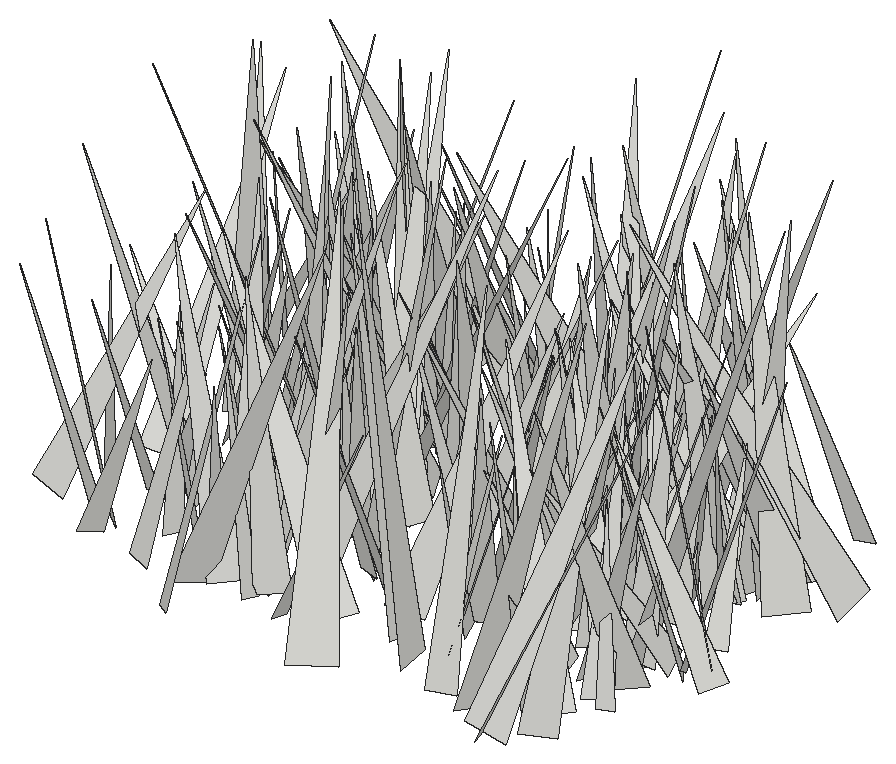
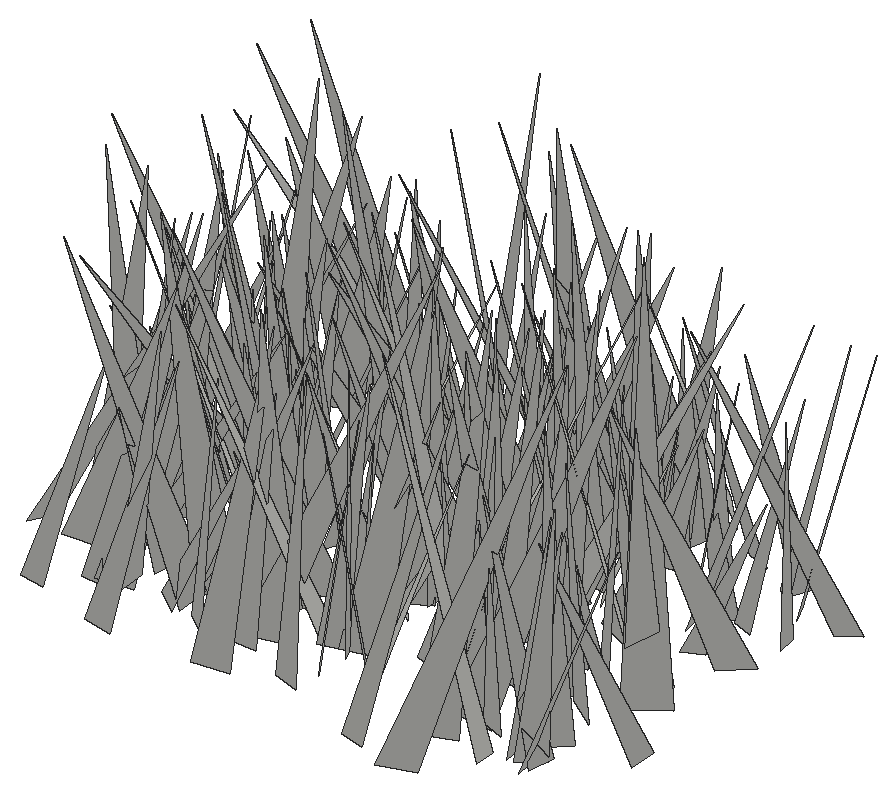
# SketchUp Ruby script. Lengths in inches.
U = 1.inch
M = Sketchup.active_model
def pt(a) = Geom::Point3d.new(a.map { |v| v * U })
def face(e, loops, mat)
  f = e.add_face(loops[0].map { |a| pt(a) })
  loops[1..].each { |l| e.add_face(l.map { |a| pt(a) }).erase! }
  f.material = f.back_material = mat if mat
  f
end
# faces: each face lists its corners as indices into pts; further lists are holes
def faces(e, pts, list, mat = nil) = list.each { |f| face(e, (f[0].is_a?(Array) ? f : [f]).map { |l| l.map { |i| pts[i] } }, mat) }
# xy, xz, yz: faces in a plane at the given z, y or x. An outline is a flat list of corners, or four numbers for a rectangle; further outlines are holes
def ring(l) = l.size == 4 ? [[l[0], l[1]], [l[2], l[1]], [l[2], l[3]], [l[0], l[3]]] : l.each_slice(2).to_a
def flat(e, list, mat, &to3) = list.each { |f| face(e, (f[0].is_a?(Array) ? f : [f]).map { |l| ring(l).map { |u, v| to3.(u, v) } }, mat) }
def xy(e, z, list, mat = nil) = flat(e, list, mat) { |x, y| [x, y, z] }
def xz(e, y, list, mat = nil) = flat(e, list, mat) { |x, z| [x, y, z] }
def yz(e, x, list, mat = nil) = flat(e, list, mat) { |y, z| [x, y, z] }
def lines(e, pts, list) = list.each { |a, b| e.add_line(pt(pts[a]), pt(pts[b])) }
# prism: a flat outline (further loops are holes) pulled along v
def prism(e, loops, v, mat = nil)
  f = face(e, loops, mat); d = Geom::Vector3d.new(v.map { |x| x * U })
  f.pushpull(f.normal.samedirection?(d) ? d.length : -d.length)
end
def box(e, o, s, mat = nil) = prism(e, [[o, [o[0] + s[0], o[1], o[2]], [o[0] + s[0], o[1] + s[1], o[2]], [o[0], o[1] + s[1], o[2]]]], [0, 0, s[2]], mat)
def at(x, y, z, deg = 0) = Geom::Transformation.translation(pt([x, y, z])) * Geom::Transformation.rotation(ORIGIN, Z_AXIS, deg.degrees)
def axes(o, x, y, z) = Geom::Transformation.new([*x, 0, *y, 0, *z, 0, *pt(o).to_a, 1])
def part(name) = M.definitions.add(name)
# library, detail: a bought-in or finely detailed component or shape, given as its bounding box
def library(name, o, s) = part(name).tap { |d| box(d.entities, o, s) }
def detail(e, o, s) = box(e.add_group.entities, o, s)
def put(e, d, t, mat = nil) = e.add_instance(d, t).tap { |i| i.material = mat if mat }
def group(e, t, mat = nil) = e.add_group.tap { |g| g.transformation = t; g.material = mat if mat }.entities
root = M.entities
c1 = part("fur_instance\#9")
p = [[0.8125,0,1.79],[0.67,-0.02,1.48],[0,-0.11,0],[0,0.11,0]]
faces(c1.entities,p,[[0,1,2,3]])
put(root,c1,axes([131.79,358.97,-27.1],[7.44072,-1.6859,2.03296],[-2.09272,-7.4711,1.46382],[-1.61112,1.91833,7.48758]))
put(root,c1,axes([133.125,357.88,-27.1],[-0.55252,7.61083,1.2014],[7.43516,0.84266,-1.91879],[2.02152,-1.01911,7.38568]))
put(root,c1,axes([134.1875,358.99,-27.1],[-5.16392,-1.1559,0.80889],[-1.35151,4.93357,-1.57791],[0.40477,1.72635,5.05098]))
put(root,c1,axes([125.68,357.83,-27.1],[-5.56313,6.05819,1.00831],[6.02083,5.64819,-0.71719],[1.2116,-0.25113,8.19364]))
put(root,c1,axes([114.08,360.4,-27.1],[3.45367,-2.54495,0.42724],[-2.57712,-3.36456,0.79082],[0.1334,0.88889,4.21654]))
put(root,c1,axes([123.74,360.28,-27.1],[6.28963,-0.96384,2.1084],[-1.07131,-6.61487,0.17192],[-2.05588,0.49827,6.36073]))
put(root,c1,axes([118.91,359.8,-27.1],[6.76451,-3.26106,1.25254],[-3.47694,-6.54929,1.72622],[-0.33809,2.1058,7.30844]))
put(root,c1,axes([128.125,360.22,-27.1],[-7.87878,-1.52664,2.20407],[-1.70967,8.13085,-0.47967],[2.06533,0.90687,8.01097]))
put(root,c1,axes([133.12,357.53,-27.1],[6.18332,3.30926,0.01495],[3.17233,-5.93637,1.96995],[-0.9422,1.73008,6.73082]))
put(root,c1,axes([122.71,359.79,-27.1],[3.9235,0.14114,0.37721],[0.06723,-3.8717,0.74932],[-0.3971,0.73898,3.85386]))
put(root,c1,axes([119.34,357.74,-27.1],[4.35483,5.04158,0.80125],[4.65214,-4.35304,2.10539],[-2.1017,0.81089,6.32055]))
put(root,c1,axes([118.79,361.35,-27.1],[3.85883,-1.0172,1.02296],[-0.87371,-3.97244,-0.65425],[-1.14794,-0.39587,3.93665]))
put(root,c1,axes([113.28,361.72,-27.1],[-4.38014,-2.49103,0.91186],[-2.44951,4.47381,0.4553],[1.01814,0.04674,5.01832]))
put(root,c1,axes([129.71,359.67,-27.1],[2.50571,3.8301,0.73521],[3.84486,-2.57244,0.29737],[-0.65369,-0.44905,4.56726]))
put(root,c1,axes([121.5625,360.86,-27.1],[-3.51075,4.42455,2.16586],[4.8357,3.60279,0.47842],[0.94002,-2.00904,5.62789]))
put(root,c1,axes([119.84,360.53,-27.1],[-3.34146,5.15286,1.47209],[5.35695,3.16362,1.08579],[-0.14849,-1.82317,6.0447]))
put(root,c1,axes([116.61,359.82,-27.1],[2.03381,4.83721,0.83738],[4.90479,-2.04045,-0.1258],[-0.20703,-0.82108,5.24587]))
put(root,c1,axes([121.15,360.2,-27.1],[-4.31173,0.11749,0.33288],[0.02447,4.16916,-1.1546],[0.35215,1.14887,4.15592]))
put(root,c1,axes([114.28,361.38,-27.1],[-4.01169,-3.78695,1.3287],[-4.00574,3.89344,-0.9976],[0.2459,1.64323,5.42581]))
put(root,c1,axes([125.25,362.83,-27.1],[-2.82637,-5.01502,0.69558],[-5.06125,2.81969,-0.23605],[0.13409,0.7222,5.75179]))
put(root,c1,axes([132.3,360.89,-27.1],[-3.8319,-0.08961,1.0116],[-0.27638,3.8917,-0.7022],[0.97723,0.7493,3.76807]))
put(root,c1,axes([134.18,360.33,-27.1],[-3.78417,5.30239,0.2634],[5.25954,3.70033,1.07214],[-0.72248,-0.83479,6.42541]))
put(root,c1,axes([124.35,360.86,-27.1],[-4.44973,5.42889,0.1833],[5.21151,4.19987,2.12315],[-1.53186,-1.48148,6.69068]))
put(root,c1,axes([135.0625,363.33,-27.1],[2.07945,-5.56592,1.40736],[-5.43571,-2.39045,-1.42237],[-1.84751,0.76846,5.76892]))
put(root,c1,axes([130.25,359.08,-27.1],[0.51601,7.02264,0.2402],[6.84431,-0.55684,1.57697],[-1.5908,-0.11784,6.86272]))
put(root,c1,axes([120.35,361.39,-27.1],[0.83525,-3.69964,2.10924],[-4.22949,-0.46947,0.8514],[0.49764,2.21949,3.69595]))
put(root,c1,axes([118.83,362.11,-27.1],[-2.76713,3.18046,1.2921],[3.43249,2.58898,0.97827],[0.05304,-1.61979,4.10065]))
put(root,c1,axes([134.68,358.78,-27.1],[-6.77077,3.15469,0.89527],[2.64884,6.47215,-2.77341],[1.93319,2.18084,6.93567]))
put(root,c1,axes([117.28,362.17,-27.1],[-3.57369,-1.9669,1.0397],[-2.0892,3.64317,-0.28897],[0.76478,0.76131,4.06896]))
put(root,c1,axes([128.33,363.02,-27.1],[-3.2792,-1.26365,1.37089],[-0.97388,3.52607,0.9207],[1.58988,-0.44645,3.3915]))
put(root,c1,axes([128.36,363.73,-27.1],[2.49567,-4.97649,0.70111],[-5.02561,-2.47346,0.33254],[-0.01412,0.77585,5.55727]))
put(root,c1,axes([120.59,361.31,-27.1],[4.03025,7.20792,1.49357],[7.34455,-3.82368,-1.36555],[0.49235,-1.96292,8.14446]))
put(root,c1,axes([126.84,361.29,-27.1],[-7.00273,-0.39667,0.95685],[-0.59042,6.90153,-1.45992],[0.85107,1.52402,6.86034]))
put(root,c1,axes([116.36,362.03,-27.1],[-3.76859,1.24193,1.36163],[1.17189,4.00702,-0.41131],[1.42236,-0.01087,3.94658]))
put(root,c1,axes([114.88,363.66,-27.1],[1.3305,-3.93215,0.09517],[-3.71952,-1.22514,1.38031],[1.27907,0.52755,3.91494]))
put(root,c1,axes([135.32,361.63,-27.1],[-0.19051,3.61425,0.52762],[3.57644,0.0773,0.76192],[-0.74175,-0.55561,3.53816]))
put(root,c1,axes([132.47,363.39,-27.1],[-4.25232,-1.15186,0.17503],[-1.13335,4.24309,0.38907],[0.27009,-0.33025,4.38835]))
put(root,c1,axes([114.16,363.74,-27.1],[-1.28236,-4.10189,0.60594],[-4.14572,1.27987,-0.10961],[0.07509,0.61118,4.29626]))
put(root,c1,axes([133.57,363.1,-27.1],[4.86131,-2.02952,0.59697],[-2.06386,-4.87843,0.22145],[-0.46454,0.43544,5.26329]))
put(root,c1,axes([119.67,361.91,-27.1],[-2.53684,6.34204,1.9532],[6.60869,2.60398,0.12835],[0.60133,-1.86275,6.82939]))
put(root,c1,axes([120.46,362.1,-27.1],[3.86814,-0.78573,1.02615],[-1.07279,-3.75781,1.16655],[-0.72076,1.37634,3.77081]))
put(root,c1,axes([135.16,365.58,-27.1],[-5.02387,-1.18033,0.42976],[-0.88594,4.58548,2.23734],[0.8905,-2.09699,4.65046]))
put(root,c1,axes([128.69,361.59,-27.1],[4.75922,3.00167,0.77273],[2.8511,-4.79497,1.06623],[-1.21588,0.50555,5.5248]))
put(root,c1,axes([128.02,364.64,-27.1],[6.9866,-0.46387,0.39437],[-0.38095,-6.874,-1.33651],[-0.47495,-1.31005,6.87325]))
put(root,c1,axes([111.05,361.9,-27.1],[0.65701,6.39206,0.99008],[6.12037,-0.29236,-2.17392],[2.09278,-1.15171,6.04683]))
put(root,c1,axes([134.65,362.01,-27.1],[-3.96377,3.38106,0.80717],[3.27975,4.04327,-0.83051],[1.15166,0.12228,5.14327]))
put(root,c1,axes([120.79,364.92,-27.1],[2.81621,-4.35059,0.38195],[-4.36621,-2.81499,0.12899],[-0.09891,0.39082,5.18093]))
put(root,c1,axes([112.28,363.67,-27.1],[3.8396,0.83392,1.68617],[0.96833,-4.16197,-0.14664],[-1.61273,-0.51356,3.92638]))
put(root,c1,axes([123.21,364,-27.1],[-3.81075,-5.76969,1.72606],[-6.01138,3.52106,-1.50194],[-0.36316,2.25903,6.74947]))
put(root,c1,axes([115.74,364.3,-27.1],[-6.60705,-1.5953,0.55499],[-1.61141,6.62494,-0.14037],[0.50631,0.26714,6.79547]))
put(root,c1,axes([135.77,365.24,-27.1],[-4.16981,-3.31895,0.85743],[-3.36405,4.22145,-0.01946],[0.65859,0.54939,5.32938]))
put(root,c1,axes([122.56,361.57,-27.1],[3.274,7.7332,0.0389],[7.72076,-3.26624,-0.49451],[0.44025,-0.22856,8.38313]))
put(root,c1,axes([130.0625,362.83,-27.1],[4.92859,0.75105,0.39032],[0.57555,-4.66461,1.7081],[-0.62062,1.63853,4.68375]))
put(root,c1,axes([130.85,365.08,-27.1],[4.88822,-0.89007,0.63341],[-0.87396,-4.92864,-0.18113],[-0.65546,-0.06625,4.96529]))
put(root,c1,axes([137.24,365.07,-27.1],[-3.88127,2.88585,0.74535],[2.95869,3.58243,1.53633],[-0.36036,-1.66913,4.58608]))
put(root,c1,axes([117.11,365.25,-27.1],[-3.35519,-0.75879,1.11745],[-0.66434,3.53232,0.40387],[1.17606,-0.1694,3.41613]))
put(root,c1,axes([122.875,364.34,-27.1],[4.94057,6.27292,2.28459],[6.62263,-4.9638,-0.69253],[-0.84236,-2.23369,7.95482]))
put(root,c1,axes([121.28,365.89,-27.1],[4.3252,-1.84495,1.08949],[-1.74272,-4.45705,-0.62914],[-1.2465,-0.1704,4.65998]))
put(root,c1,axes([119.76,364.64,-27.1],[-1.17344,-6.36654,3.3674],[-7.15717,1.41187,0.17527],[0.80444,3.27459,6.4714]))
put(root,c1,axes([133.66,363.99,-27.1],[-3.54308,4.52564,0.44169],[4.5332,3.47169,0.79207],[-0.35583,-0.83417,5.69276]))
put(root,c1,axes([119.19,364.98,-27.1],[-3.56795,-1.90054,0.20659],[-1.88749,3.43261,-1.0196],[-0.30353,0.99505,3.91187]))
put(root,c1,axes([121.06,365.91,-27.1],[3.12862,-2.29976,0.97047],[-2.27,-3.26853,-0.42753],[-1.03819,0.21622,3.85932]))
put(root,c1,axes([119.6,366.09,-27.1],[-2.97,-5.19915,0.68344],[-5.09037,2.66981,-1.8109],[-1.25951,1.46972,5.70725]))
put(root,c1,axes([134.15,364.83,-27.1],[-0.55684,5.82392,2.02647],[6.12632,0.75415,-0.48394],[0.70204,-1.96161,5.83043]))
put(root,c1,axes([126.51,365.66,-27.1],[-4.66446,-0.17714,0.77084],[-0.14932,4.72517,0.1823],[0.77671,-0.15541,4.66426]))
put(root,c1,axes([135.9,366.5625,-27.1],[4.20893,3.73459,3.7879],[4.59902,-4.98198,-0.19834],[-2.67289,-2.69131,5.62342]))
put(root,c1,axes([131.53,367.64,-27.1],[4.41778,-6.32124,1.65754],[-6.32459,-4.6393,-0.83587],[-1.6447,0.86086,7.66656]))
put(root,c1,axes([124.6,366.7,-27.1],[3.18493,-3.37138,0.77047],[-3.44968,-3.17103,0.3845],[-0.24394,0.82581,4.62191]))
put(root,c1,axes([132.14,364.63,-27.1],[-4.57761,1.25738,1.06742],[0.91701,4.55759,-1.43608],[1.37093,1.14988,4.52473]))
put(root,c1,axes([131.1,365.93,-27.1],[1.65832,3.59632,1.35209],[3.82471,-1.68517,-0.20869],[-0.36513,-1.31848,3.95475]))
put(root,c1,axes([125.84,362.64,-27.1],[-5.17652,4.83446,1.05401],[3.91261,4.93311,-3.41105],[3.02894,1.88989,6.20751]))
put(root,c1,axes([114.41,366.1,-27.1],[-3.16167,2.60611,0.16715],[2.5519,3.02748,1.0668],[-0.55458,-0.92652,3.956]))
put(root,c1,axes([118.93,368.58,-27.1],[7.2919,-1.58164,0.56037],[-1.39543,-7.10365,-1.89164],[-0.93186,-1.73896,7.21769]))
put(root,c1,axes([129.96,366.41,-27.1],[-5.05494,-2.22544,0.30278],[-2.23904,4.935,-1.10864],[-0.17591,1.1357,5.41072]))
put(root,c1,axes([127.45,368.08,-27.1],[-5.15654,-2.89646,0.02201],[-2.88562,5.14083,0.47427],[0.2514,-0.40276,5.89529]))
put(root,c1,axes([131.22,365.33,-27.1],[-1.86481,4.13252,0.34952],[4.14724,1.85655,0.17621],[-0.01744,-0.39104,4.53037]))
put(root,c1,axes([130.72,367.17,-27.1],[4.45339,-2.56263,0.11815],[-2.55046,-4.39735,0.75645],[0.27609,0.71411,5.08208]))
put(root,c1,axes([119.44,367.03,-27.1],[-6.03257,-5.76703,0.56772],[-5.59645,5.58532,-2.7307],[-1.50355,2.34912,7.8863]))
put(root,c1,axes([128.52,368.02,-27.1],[-4.47409,-0.55232,0.95951],[-0.288,4.43762,1.21151],[1.069,-1.11608,4.34221]))
put(root,c1,axes([119.45,366.52,-27.1],[5.54301,-4.89223,1.08245],[-4.92161,-5.01325,2.54471],[0.93987,2.60075,6.94141]))
put(root,c1,axes([132.03,368.08,-27.1],[-2.90046,-3.39812,1.38689],[-3.27993,3.19309,0.96417],[1.64705,0.37459,4.36237]))
put(root,c1,axes([133.33,366.18,-27.1],[-4.45117,0.87592,1.04433],[0.68712,4.52233,-0.86441],[1.17717,0.67238,4.45342]))
put(root,c1,axes([117.28,366.79,-27.1],[-0.49335,5.1966,1.87912],[5.02115,-0.36617,2.33091],[-2.30734,-1.90798,4.67065]))
put(root,c1,axes([134.33,364.45,-27.1],[7.79418,1.63756,2.08164],[0.8535,-7.67768,2.8441],[-2.50726,2.47704,7.43922]))
put(root,c1,axes([123.875,369.34,-27.1],[4.30968,-5.09044,0.61484],[-5.06109,-4.35201,-0.55619],[-0.82219,0.10671,6.64655]))
put(root,c1,axes([113.53,368.77,-27.1],[6.27835,0.76334,0.54412],[0.88551,-6.03847,-1.74618],[-0.30762,-1.80294,6.07875]))
put(root,c1,axes([116.91,369.44,-27.1],[-0.2881,-6.79413,1.19024],[-6.52945,0.65262,2.14482],[2.22333,1.03623,6.45314]))
put(root,c1,axes([130.15,368.46,-27.1],[-3.55733,-3.55392,1.20149],[-3.66341,3.64755,-0.05732],[0.80828,0.89081,5.02808]))
put(root,c1,axes([114.26,368.78,-27.1],[1.4923,-4.43759,0.64343],[-4.35505,-1.27294,1.3215],[1.06759,1.01025,4.49142]))
put(root,c1,axes([118.21,367.39,-27.1],[3.92442,2.27765,0.90763],[2.32456,-4.0011,-0.01041],[-0.77966,-0.46478,4.53747]))
put(root,c1,axes([129.31,368.47,-27.1],[1.81609,-4.28388,1.69446],[-4.45246,-2.09973,-0.53642],[-1.18256,1.32684,4.62191]))
put(root,c1,axes([131.38,366.43,-27.1],[7.46967,2.68884,2.29218],[2.3982,-7.79505,1.32883],[-2.59473,0.53597,7.82688]))
put(root,c1,axes([124.96,367.39,-27.1],[0.90877,4.85728,1.17196],[4.86719,-0.59112,-1.32422],[1.13009,-1.36012,4.76083]))
put(root,c1,axes([122.35,367.67,-27.1],[-5.92125,2.00992,1.02968],[2.02644,6.00419,-0.06686],[0.99676,-0.26678,6.25272]))
put(root,c1,axes([135.64,367.19,-27.1],[-2.23531,2.8422,0.49749],[2.78374,2.28983,-0.57415],[0.75919,-0.0278,3.57002]))
put(root,c1,axes([135.74,365.3,-27.1],[4.27823,3.00126,0.70858],[2.21616,-3.83495,2.86263],[-2.14435,2.02448,4.3722]))
put(root,c1,axes([131.73,367.75,-27.1],[5.13146,2.31605,0.71954],[2.33013,-5.17519,0.0403],[-0.67253,-0.25897,5.62978]))
put(root,c1,axes([121.19,370.19,-27.1],[-6.73685,-3.71008,0.0403],[-3.70619,6.73292,0.28887],[0.17463,-0.23362,7.68547]))
put(root,c1,axes([123.37,368.46,-27.1],[5.69837,-0.41307,2.53776],[-0.52377,-6.22748,0.16244],[-2.51724,0.36068,5.71101]))
put(root,c1,axes([133.03,369.15,-27.1],[4.02483,1.17033,1.17041],[1.40502,-4.04247,-0.78939],[-0.87491,-1.10794,4.11653]))
put(root,c1,axes([134.375,369.09,-27.1],[-3.74193,-1.93414,1.83822],[-1.95383,4.14237,0.38123],[1.81727,0.47108,4.19495]))
put(root,c1,axes([131.4,368.625,-27.1],[1.02394,3.35387,1.44831],[3.57422,-1.23084,0.32333],[-0.75567,-1.27715,3.49176]))
put(root,c1,axes([112.5625,366.07,-27.1],[-2.48989,6.58556,0.19317],[6.42005,2.47161,-1.51018],[1.47984,0.3578,6.87667]))
put(root,c1,axes([113.17,370.14,-27.1],[4.71718,-6.41333,2.08506],[-6.64537,-4.85367,0.10513],[-1.14777,1.74389,7.96063]))
put(root,c1,axes([113.81,369.82,-27.1],[4.65785,-0.69082,1.21899],[-0.53967,-4.78978,-0.65231],[-1.29303,-0.48941,4.6634]))
put(root,c1,axes([133.98,369.73,-27.1],[4.51203,-4.20905,2.90182],[-4.30887,-5.21386,-0.8628],[-2.75143,1.26279,6.10984]))
put(root,c1,axes([119.36,370,-27.1],[-4.57691,0.82768,1.57562],[1.18388,4.66198,0.99001],[1.32893,-1.30255,4.54457]))
put(root,c1,axes([115.57,369.44,-27.1],[-3.42106,-4.15596,2.05732],[-4.44833,3.66341,0.00339],[1.31032,1.58608,5.3829]))
put(root,c1,axes([133.96,370.01,-27.1],[0.76269,-3.95415,0.89534],[-4.04548,-0.80213,-0.09639],[-0.26648,0.86018,4.02588]))
put(root,c1,axes([114.61,370.36,-27.1],[5.46808,5.3055,1.78388],[5.41419,-4.38056,-3.56761],[1.42026,-3.72732,6.73205]))
put(root,c1,axes([116.31,367.18,-27.1],[-5.10797,-4.03263,5.02727],[-5.71036,5.80586,-1.14484],[2.98787,4.202,6.40647]))
put(root,c1,axes([126.93,369.03,-27.1],[3.29579,4.51514,1.8086],[4.80118,-3.36974,-0.33663],[-0.7786,-1.66678,5.57991]))
put(root,c1,axes([115.91,371.3,-27.1],[6.82649,-0.20783,2.36031],[0.47416,-6.93274,-1.9818],[-2.32152,-2.02711,6.5358]))
put(root,c1,axes([129.52,368.7,-27.1],[-4.01098,-1.65554,1.8183],[-2.11594,4.09606,-0.93811],[1.25294,1.61753,4.23659]))
put(root,c1,axes([117.26,370.38,-27.1],[4.37094,-3.26497,1.75227],[-3.26747,-4.6741,-0.55863],[-1.74761,0.57306,5.42707]))
put(root,c1,axes([119.2,371.88,-27.1],[1.9027,-5.40071,0.1352],[-5.35593,-1.9045,-0.70218],[-0.70705,-0.10684,5.68285]))
put(root,c1,axes([134.92,372.22,-27.1],[3.41213,-4.67618,0.33772],[-4.46229,-3.36731,-1.54031],[-1.43828,-0.64649,5.58003]))
put(root,c1,axes([129.73,370.9,-27.1],[4.8829,2.83209,2.83107],[3.60518,-5.05239,-1.16384],[-1.7431,-2.51617,5.52349]))
put(root,c1,axes([119.6,372.35,-27.1],[-3.6044,-3.37024,0.34721],[-3.01204,3.4196,1.92476],[1.55135,-1.19103,4.54373]))
put(root,c1,axes([120.65,368.83,-27.1],[7.61599,0.93725,0.32253],[0.89381,-7.57423,0.90437],[-0.42844,0.85927,7.61996]))
put(root,c1,axes([131.21,367.11,-27.1],[-1.51427,6.54379,0.36236],[5.84338,1.51647,-2.96661],[2.96773,0.35306,6.02606]))
put(root,c1,axes([133.4,367.65,-27.1],[1.19903,6.87384,0.5978],[6.78552,-1.2847,1.16229],[-1.25048,-0.38022,6.88014]))
put(root,c1,axes([121.6,366.96,-27.1],[-6.67493,4.02137,0.12146],[3.83511,6.43107,-2.16198],[1.21576,1.79188,7.48679]))
put(root,c1,axes([127.54,370.84,-27.1],[3.13574,-5.33007,1.5739],[-5.55752,-3.01682,0.85589],[-0.02918,1.79133,6.12454]))
put(root,c1,axes([118.34,371.53,-27.1],[-1.31696,-6.51866,1.83434],[-6.75362,1.40125,0.13086],[0.49623,1.77078,6.64907]))
put(root,c1,axes([137.375,372.46,-27.1],[-8.16776,0.06376,0.0825],[0.08376,7.86119,2.21763],[0.06209,-2.2183,7.8612]))
put(root,c1,axes([130.9,368.74,-27.1],[-2.1836,4.82414,0.14178],[4.82373,2.17653,0.23433],[-0.15514,-0.2257,5.29014]))
put(root,c1,axes([123.6875,370.83,-27.1],[-2.7685,-2.84273,0.0732],[-2.6967,2.59213,-1.32656],[-0.90237,0.97511,3.73978]))
put(root,c1,axes([123.1,373.09,-27.1],[2.89826,-6.60565,0.55734],[-6.55377,-2.94663,-0.84295],[-0.99662,0.16719,7.16407]))
put(root,c1,axes([125.18,371.19,-27.1],[4.42222,0.57042,2.59632],[0.96066,-5.04183,-0.52855],[-2.47858,-0.93641,4.42741]))
put(root,c1,axes([119.11,372.31,-27.1],[8.07507,1.50255,0.4439],[1.56674,-7.73574,-2.31627],[0.00564,-2.35841,7.88031]))
put(root,c1,axes([123.63,369.97,-27.1],[4.56915,3.9518,0.34933],[3.96081,-4.51383,-0.74378],[0.22516,-0.79028,5.99505]))
put(root,c1,axes([135.98,370.56,-27.1],[-4.89648,5.17695,2.06152],[5.4889,4.95404,0.59637],[0.96057,-1.91907,7.10075]))
put(root,c1,axes([125.12,369.69,-27.1],[-0.69382,4.82103,0.91338],[4.82167,0.84094,-0.77604],[0.90996,-0.78004,4.80848]))
put(root,c1,axes([114.05,369.16,-27.1],[-5.08982,4.44528,0.70369],[4.40622,5.13821,-0.58816],[0.91699,-0.01575,6.73207]))
put(root,c1,axes([132.63,374.53,-27.1],[4.86562,-4.5964,0.06859],[-4.19123,-4.47675,-2.68294],[-1.88818,-1.90726,6.13213]))
put(root,c1,axes([124.48,371.76,-27.1],[-4.64353,0.24048,0.81476],[0.40253,4.60984,0.93348],[0.74809,-0.98772,4.55508]))
put(root,c1,axes([117.37,374.41,-27.1],[2.70234,-6.75975,0.1599],[-6.39067,-2.60962,-2.31767],[-2.20886,-0.71979,6.90111]))
put(root,c1,axes([121.1875,368.74,-27.1],[-7.30125,2.0292,0.54339],[1.84392,7.1322,-1.85816],[1.00641,1.65384,7.34664]))
put(root,c1,axes([126.63,371.87,-27.1],[3.82304,5.79974,2.60132],[6.29108,-3.01834,-2.51622],[0.9089,-3.50316,6.47466]))
put(root,c1,axes([133.48,371.84,-27.1],[-5.14523,1.96025,0.06602],[1.88898,4.90265,1.64806],[-0.52792,-1.56261,5.25356]))
put(root,c1,axes([134.15,371.11,-27.1],[6.73151,-1.98165,2.55494],[-2.23492,-7.11595,0.36912],[-2.33662,1.09735,7.00742]))
put(root,c1,axes([119.16,371.98,-27.1],[5.28351,-1.61661,1.62366],[-1.56193,-5.52709,-0.42043],[-1.67632,0.05465,5.50927]))
put(root,c1,axes([120.97,372.27,-27.1],[-0.75955,-3.70224,0.74684],[-3.72635,0.61048,-0.76351],[-0.61539,0.87293,3.70143]))
put(root,c1,axes([125.07,370.55,-27.1],[-3.90269,-1.36809,1.23152],[-1.73858,3.68797,-1.41263],[0.60468,1.77384,3.88679]))
put(root,c1,axes([119.1,371.35,-27.1],[4.24793,5.0228,3.04998],[5.34423,-4.86703,0.57187],[-2.44337,-1.91294,6.55335]))
put(root,c1,axes([120.46,368.7,-27.1],[-0.64935,7.68845,0.01437],[7.6155,0.6412,1.06165],[-1.05669,-0.10353,7.64243]))
put(root,c1,axes([134.51,371.29,-27.1],[-6.69372,-1.63538,1.73187],[-1.91789,6.76382,-1.02573],[1.41263,1.43387,6.81383]))
put(root,c1,axes([126.54,374.4,-27.1],[-6.66712,2.68909,2.42043],[3.53397,5.92752,3.14894],[0.77508,-3.89533,6.46266]))
put(root,c1,axes([130.28,369.51,-27.1],[5.47327,5.90798,0.9862],[5.7796,-5.55993,1.23167],[-1.57262,0.12835,7.95889]))
put(root,c1,axes([128.42,371.91,-27.1],[4.16572,3.95636,0.93283],[4.06431,-4.03236,-1.04767],[0.06588,-1.40123,5.64875]))
put(root,c1,axes([120.16,371.75,-27.1],[1.76175,3.91399,1.38102],[4.01071,-1.99148,0.5277],[-1.06803,-1.02224,4.25965]))
put(root,c1,axes([113.99,373.96,-27.1],[4.00821,-3.73033,0.31245],[-3.73197,-4.01777,-0.09299],[-0.29215,0.14465,5.47471]))
put(root,c1,axes([124.15,373.37,-27.1],[1.70929,-4.46495,1.67991],[-4.63149,-1.98085,-0.55231],[-1.1433,1.34907,4.74893]))
put(root,c1,axes([132.97,374.89,-27.1],[-0.03159,-6.8611,0.78211],[-6.88005,-0.03586,-0.59249],[-0.59273,0.78192,6.83555]))
put(root,c1,axes([114.78,371.66,-27.1],[2.34142,5.16985,1.64131],[5.10687,-2.70355,1.23051],[-1.82787,-0.93109,5.54034]))
put(root,c1,axes([126.36,370.72,-27.1],[0.38295,8.08113,1.09098],[7.9956,-0.1576,-1.6392],[1.60161,-1.14545,7.92239]))
put(root,c1,axes([123.53,373.23,-27.1],[-4.21315,-2.34987,2.26772],[-2.4638,4.71684,0.31027],[2.14339,0.80291,4.81418]))
put(root,c1,axes([129.85,372.48,-27.1],[-6.207,1.9177,0.03314],[1.91765,6.20287,0.22937],[-0.03607,-0.22893,6.49244]))
put(root,c1,axes([117.54,375.99,-27.1],[2.10072,-7.09935,0.00934],[-7.09522,-2.09917,0.25546],[0.24231,0.08144,7.39923]))
put(root,c1,axes([129.44,372.92,-27.1],[3.63637,-5.76719,3.12725],[-6.51934,-3.57646,0.98508],[-0.73369,3.19558,6.74635]))
put(root,c1,axes([111.13,372.89,-27.1],[4.26787,-0.90452,0.30078],[-0.95208,-4.11231,1.14272],[-0.04649,1.18073,4.21035]))
put(root,c1,axes([130.48,374.4,-27.1],[-2.43952,-3.83837,0.4143],[-3.75379,2.24378,-1.31547],[-0.90209,1.04325,4.3536]))
put(root,c1,axes([123.49,374.89,-27.1],[-3.34648,-2.86729,1.25208],[-2.75468,3.56945,0.81158],[1.4835,0.16004,4.33146]))
put(root,c1,axes([135.27,372.89,-27.1],[-3.78872,6.01371,0.63065],[5.87535,3.48538,2.06137],[-1.42923,-1.61377,6.8022]))
put(root,c1,axes([131.91,372.57,-27.1],[-3.54385,2.2292,0.7922],[1.93522,3.55225,-1.33876],[1.36083,0.75365,3.96686]))
put(root,c1,axes([127.14,372.6,-27.1],[-5.31707,5.30249,0.96243],[5.27581,5.39738,-0.58989],[1.09932,-0.2564,7.48596]))
put(root,c1,axes([113.87,375.93,-27.1],[-4.07009,-1.55263,0.42821],[-1.43545,4.0247,0.94922],[0.73043,-0.7422,4.25151]))
put(root,c1,axes([114.78,374.67,-27.1],[-3.50037,2.65675,1.28484],[2.86731,3.53339,0.50538],[0.69832,-1.19104,4.36526]))
put(root,c1,axes([129.83,373.64,-27.1],[7.1879,-0.3196,1.18159],[-0.53762,-7.14753,1.33717],[-1.09967,1.40532,7.06966]))
put(root,c1,axes([126.66,375.14,-27.1],[0.55696,-4.64877,2.01019],[-4.98122,-0.86859,-0.62855],[-0.91614,1.89648,4.63963]))
put(root,c1,axes([134.92,376.12,-27.1],[0.09538,-4.31944,0.7575],[-4.29634,-0.24392,-0.84995],[-0.8791,0.72346,4.23607]))
put(root,c1,axes([128.7,375.01,-27.1],[2.49829,3.83803,2.30798],[4.11646,-3.0089,0.54773],[-1.76409,-1.58579,4.54664]))
put(root,c1,axes([115.36,376.125,-27.1],[6.89965,2.05968,0.48381],[2.11498,-6.67017,-1.76557],[0.05673,-1.82978,6.98071]))
put(root,c1,axes([113.62,375.25,-27.1],[4.85484,-0.93426,0.93937],[-1.01134,-4.91828,0.33525],[-0.85583,0.51221,4.93253]))
put(root,c1,axes([116.41,374.43,-27.1],[0.5097,3.85536,0.87755],[3.83119,-0.70034,0.85159],[-0.9777,-0.73445,3.79452]))
put(root,c1,axes([114.83,375.09,-27.1],[-5.03296,-0.41167,1.23228],[-0.52474,5.15421,-0.42127],[1.18855,0.5323,5.03216]))
put(root,c1,axes([119.65,377.94,-27.1],[-2.17037,-5.72704,0.1674],[-5.69455,2.17595,0.61228],[0.63178,-0.0613,6.09382]))
put(root,c1,axes([125.42,372.32,-27.1],[6.25178,5.32919,0.93445],[4.93149,-6.20008,2.36594],[-2.22574,1.23164,7.86685]))
put(root,c1,axes([119.88,377.53,-27.1],[-3.92471,-3.72483,0.22437],[-3.66233,3.90735,0.80501],[0.71557,-0.43166,5.35067]))
put(root,c1,axes([114.01,375.31,-27.1],[3.17127,-3.30736,3.04126],[-3.82504,-3.9403,-0.2965],[-2.35731,1.94429,4.57249]))
put(root,c1,axes([121.37,374.81,-27.1],[3.52114,3.87417,1.40413],[3.91467,-3.72163,0.45161],[-1.28689,-0.72073,5.21571]))
put(root,c1,axes([123.875,376.22,-27.1],[-1.84582,-5.09705,1.94608],[-5.40108,1.99766,0.10933],[0.77171,1.78987,5.41987]))
put(root,c1,axes([117.24,378.55,-27.1],[-7.12654,1.94071,2.81889],[3.04033,6.57978,3.15641],[1.57127,-3.9294,6.67765]))
put(root,c1,axes([126.48,377.02,-27.1],[1.47343,-6.07806,1.78682],[-6.21699,-1.74005,-0.79238],[-1.21846,1.52838,6.20371]))
put(root,c1,axes([131.23,377.2,-27.1],[-0.49716,-5.04462,0.80589],[-5.07325,0.39247,-0.67299],[-0.59982,0.86174,5.02418]))
put(root,c1,axes([132.2,374.41,-27.1],[-6.81045,0.95525,0.6863],[0.79996,6.71798,-1.4123],[0.86231,1.31226,6.73054]))
